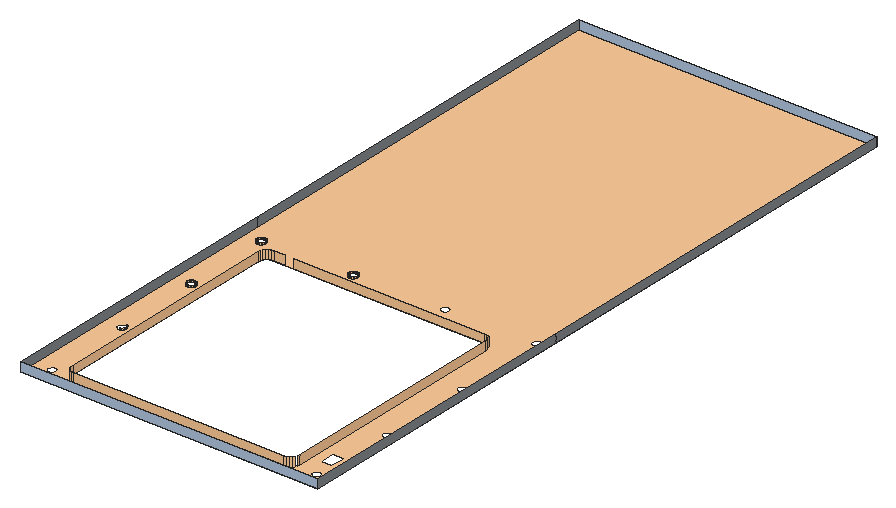
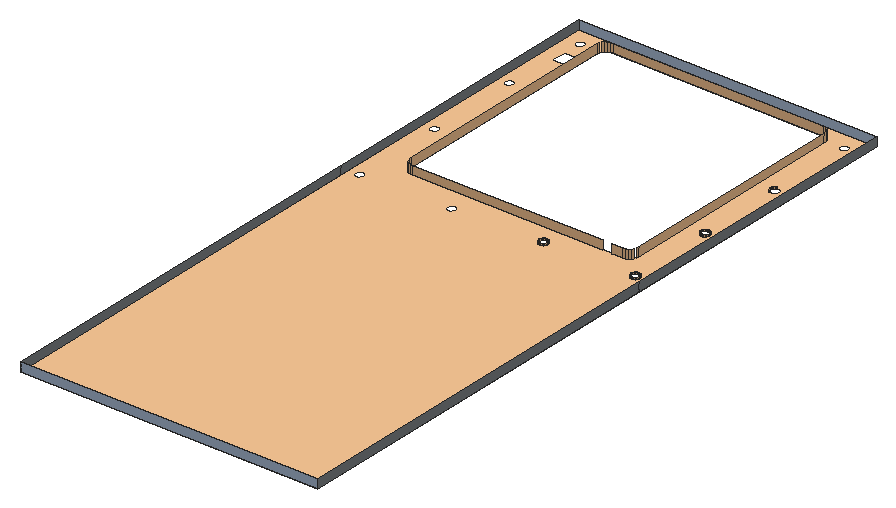
# SketchUp Ruby script. Lengths in inches.
U = 1.inch
M = Sketchup.active_model
def pt(a) = Geom::Point3d.new(a.map { |v| v * U })
def face(e, loops, mat)
  f = e.add_face(loops[0].map { |a| pt(a) })
  loops[1..].each { |l| e.add_face(l.map { |a| pt(a) }).erase! }
  f.material = f.back_material = mat if mat
  f
end
# faces: each face lists its corners as indices into pts; further lists are holes
def faces(e, pts, list, mat = nil) = list.each { |f| face(e, (f[0].is_a?(Array) ? f : [f]).map { |l| l.map { |i| pts[i] } }, mat) }
# xy, xz, yz: faces in a plane at the given z, y or x. An outline is a flat list of corners, or four numbers for a rectangle; further outlines are holes
def ring(l) = l.size == 4 ? [[l[0], l[1]], [l[2], l[1]], [l[2], l[3]], [l[0], l[3]]] : l.each_slice(2).to_a
def flat(e, list, mat, &to3) = list.each { |f| face(e, (f[0].is_a?(Array) ? f : [f]).map { |l| ring(l).map { |u, v| to3.(u, v) } }, mat) }
def xy(e, z, list, mat = nil) = flat(e, list, mat) { |x, y| [x, y, z] }
def xz(e, y, list, mat = nil) = flat(e, list, mat) { |x, z| [x, y, z] }
def yz(e, x, list, mat = nil) = flat(e, list, mat) { |y, z| [x, y, z] }
def lines(e, pts, list) = list.each { |a, b| e.add_line(pt(pts[a]), pt(pts[b])) }
# prism: a flat outline (further loops are holes) pulled along v
def prism(e, loops, v, mat = nil)
  f = face(e, loops, mat); d = Geom::Vector3d.new(v.map { |x| x * U })
  f.pushpull(f.normal.samedirection?(d) ? d.length : -d.length)
end
def box(e, o, s, mat = nil) = prism(e, [[o, [o[0] + s[0], o[1], o[2]], [o[0] + s[0], o[1] + s[1], o[2]], [o[0], o[1] + s[1], o[2]]]], [0, 0, s[2]], mat)
def at(x, y, z, deg = 0) = Geom::Transformation.translation(pt([x, y, z])) * Geom::Transformation.rotation(ORIGIN, Z_AXIS, deg.degrees)
def axes(o, x, y, z) = Geom::Transformation.new([*x, 0, *y, 0, *z, 0, *pt(o).to_a, 1])
def part(name) = M.definitions.add(name)
# library, detail: a bought-in or finely detailed component or shape, given as its bounding box
def library(name, o, s) = part(name).tap { |d| box(d.entities, o, s) }
def detail(e, o, s) = box(e.add_group.entities, o, s)
def put(e, d, t, mat = nil) = e.add_instance(d, t).tap { |i| i.material = mat if mat }
def group(e, t, mat = nil) = e.add_group.tap { |g| g.transformation = t; g.material = mat if mat }.entities
root = M.entities
M.materials.add("[0099_LightSteelBlue]").color = [176, 196, 222]
M.materials.add("[Blacktop Old 01]").color = [132, 136, 139]
M.materials.add("[Color C02]").color = [255, 204, 153]
xy(root,372,[[[0,130.0625,203.78,607.58],[30,138.625,173.78,138.625,175.61,138.79,177.11,139.29,178.28,140.125,179.11,141.29,179.61,142.79,179.78,144.625,179.78,303.17,179.61,305,179.11,306.5,178.28,307.67,177.11,308.5,175.61,309,173.78,309.17,30,309.17,28.17,309,26.67,308.5,25.5,307.67,24.67,306.5,24.17,305,24,303.17,24,144.625,24.17,142.79,24.67,141.29,25.5,140.125,26.67,139.29,28.17,138.79],[186.48,154.03,194.3,164.47],[196.29,195.4,197.07,195.47,197.81,195.74,198.45,196.19,198.95,196.78,199.29,197.49,199.42,198.27,199.36,199.05,199.09,199.78,198.64,200.42,198.04,200.93,197.33,201.26,196.56,201.4,195.78,201.33,195.04,201.0625,194.4,200.61,193.9,200.01,193.57,199.3,193.43,198.53,193.5,197.75,193.76,197.02,194.21,196.375,194.8125,195.87,195.52,195.54],[196.29,259.4,197.07,259.47,197.81,259.74,198.45,260.19,198.95,260.78,199.29,261.49,199.42,262.27,199.36,263.05,199.09,263.78,198.64,264.42,198.04,264.93,197.33,265.26,196.56,265.4,195.78,265.33,195.04,265.0625,194.4,264.61,193.9,264.01,193.57,263.3,193.43,262.53,193.5,261.75,193.76,261.02,194.21,260.375,194.8125,259.87,195.52,259.54],[193.29,138.77,194.07,138.83,194.81,139.1,195.45,139.55,195.95,140.15,196.29,140.86,196.42,141.63,196.36,142.41,196.09,143.15,195.64,143.79,195.04,144.29,194.33,144.625,193.56,144.76,192.78,144.69,192.04,144.43,191.4,143.98,190.9,143.38,190.57,142.67,190.43,141.9,190.5,141.12,190.76,140.38,191.21,139.74,191.8125,139.23,192.52,138.9],[11.87,139.23,12.65,139.3,13.38,139.57,14.02,140.02,14.53,140.62,14.86,141.33,15,142.1,14.93,142.88,14.66,143.61,14.21,144.26,13.61,144.76,12.9,145.09,12.13,145.23,11.35,145.16,10.62,144.89,9.98,144.44,9.47,143.85,9.14,143.14,9,142.36,9.07,141.58,9.34,140.85,9.79,140.21,10.39,139.7,11.1,139.37],[11.87,198.88,12.65,198.95,13.38,199.21,14.02,199.66,14.53,200.26,14.86,200.97,15,201.74,14.93,202.52,14.66,203.26,14.21,203.9,13.61,204.41,12.9,204.74,12.13,204.875,11.35,204.81,10.62,204.54,9.98,204.09,9.47,203.49,9.14,202.78,9,202.01,9.07,201.23,9.34,200.49,9.79,199.85,10.39,199.35,11.1,199.02],[11.87,258.53,12.65,258.59,13.38,258.86,14.02,259.31,14.53,259.91,14.86,260.62,15,261.39,14.93,262.17,14.66,262.91,14.21,263.55,13.61,264.05,12.9,264.38,12.13,264.52,11.35,264.45,10.62,264.19,9.98,263.74,9.47,263.14,9.14,262.43,9,261.66,9.07,260.875,9.34,260.14,9.79,259.5,10.39,258.99,11.1,258.66],[134.82,321.66,135.6,321.73,136.33,321.99,136.98,322.44,137.48,323.04,137.8125,323.75,137.95,324.52,137.88,325.3,137.61,326.04,137.16,326.68,136.56,327.18,135.86,327.52,135.08,327.65,134.3,327.58,133.57,327.32,132.93,326.87,132.42,326.27,132.09,325.56,131.95,324.79,132.02,324.01,132.29,323.27,132.74,322.63,133.34,322.125,134.05,321.79],[11.87,318.17,12.65,318.24,13.38,318.51,14.02,318.96,14.53,319.55,14.86,320.26,15,321.04,14.93,321.82,14.66,322.55,14.21,323.19,13.61,323.7,12.9,324.03,12.13,324.17,11.35,324.1,10.62,323.83,9.98,323.38,9.47,322.78,9.14,322.07,9,321.3,9.07,320.52,9.34,319.79,9.79,319.14,10.39,318.64,11.1,318.31],[73.34,319.91,74.12,319.98,74.86,320.25,75.5,320.7,76,321.3,76.34,322.01,76.47,322.78,76.4,323.56,76.14,324.29,75.6875,324.9375,75.09,325.44,74.38,325.77,73.61,325.91,72.83,325.84,72.09,325.57,71.45,325.125,70.95,324.53,70.61,323.82,70.48,323.05,70.55,322.27,70.8125,321.53,71.26,320.89,71.86,320.38,72.57,320.05],[196.29,323.4,197.07,323.47,197.81,323.74,198.45,324.19,198.95,324.78,199.29,325.49,199.42,326.27,199.36,327.05,199.09,327.78,198.64,328.42,198.04,328.93,197.33,329.26,196.56,329.4,195.78,329.33,195.04,329.0625,194.4,328.61,193.9,328.01,193.57,327.3,193.43,326.53,193.5,325.75,193.76,325.02,194.21,324.375,194.8125,323.87,195.52,323.54]]],"[Color C02]")
xz(root,130.0625,[[0,372,203.78,378]],"[0099_LightSteelBlue]")
xz(root,138.625,[[30,372,173.78,378]],"[Color C02]")
xz(root,309.17,[[30,372,37.58,378],[43.58,372,173.78,378]],"[Color C02]")
xz(root,607.58,[[0,372,203.78,378]],"[0099_LightSteelBlue]")
yz(root,0,[[130.0625,372,333.17,378],[333.17,372,607.58,378]],"[Blacktop Old 01]")
yz(root,24,[[144.625,372,303.17,378]],"[Color C02]")
yz(root,179.78,[[144.625,372,303.17,378]],"[Color C02]")
yz(root,203.78,[[130.0625,372,333.17,378],[333.17,372,607.58,378]],"[Blacktop Old 01]")
p = [[28.17,138.79,372],[28.17,138.79,378],[30,138.625,378],[30,138.625,372],[175.61,138.79,378],[175.61,138.79,372],
  [173.78,138.625,372],[173.78,138.625,378],[26.67,139.29,372],[26.67,139.29,378],[177.11,139.29,378],[177.11,139.29,372],
  [25.5,140.125,372],[25.5,140.125,378],[178.28,140.125,378],[178.28,140.125,372],[24.67,141.29,372],[24.67,141.29,378],
  [179.11,141.29,378],[179.11,141.29,372],[24,144.625,372],[24,144.625,378],[24.17,142.79,378],[24.17,142.79,372],
  [179.78,144.625,378],[179.78,144.625,372],[179.61,142.79,372],[179.61,142.79,378],[13.38,199.21,372],[12.65,198.95,372],
  [12.65,198.95,373],[13.38,199.21,373],[14.02,199.66,372],[14.02,199.66,373],[14.53,200.26,372],[14.53,200.26,373],
  [14.86,200.97,372],[14.86,200.97,373],[15,201.74,372],[15,201.74,373],[14.93,202.52,372],[14.93,202.52,373],
  [14.66,203.26,372],[14.66,203.26,373],[14.21,203.9,372],[14.21,203.9,373],[13.61,204.41,372],[13.61,204.41,373],
  [11.87,258.53,372],[11.1,258.66,372],[11.1,258.66,373],[11.87,258.53,373],[12.65,258.59,372],[12.65,258.59,373],
  [13.38,258.86,372],[13.38,258.86,373],[10.39,258.99,372],[10.39,258.99,373],[14.02,259.31,372],[14.02,259.31,373],
  [9.79,259.5,372],[9.79,259.5,373],[14.53,259.91,372],[14.53,259.91,373],[9.34,260.14,372],[9.34,260.14,373],
  [14.86,260.62,372],[14.86,260.62,373],[9.07,260.875,372],[9.07,260.875,373],[15,261.39,372],[15,261.39,373],
  [9,261.66,372],[9,261.66,373],[14.93,262.17,372],[14.93,262.17,373],[9.14,262.43,372],[9.14,262.43,373],
  [14.66,262.91,372],[14.66,262.91,373],[9.47,263.14,372],[9.47,263.14,373],[14.21,263.55,372],[14.21,263.55,373],
  [9.98,263.74,372],[9.98,263.74,373],[13.61,264.05,372],[13.61,264.05,373],[10.62,264.19,372],[10.62,264.19,373],
  [12.9,264.38,372],[12.9,264.38,373],[11.35,264.45,372],[11.35,264.45,373],[12.13,264.52,372],[12.13,264.52,373],
  [24,303.17,378],[24,303.17,372],[24.17,305,372],[24.17,305,378],[179.78,303.17,372],[179.78,303.17,378],
  [179.61,305,378],[179.61,305,372],[24.67,306.5,378],[24.67,306.5,372],[25.5,307.67,372],[25.5,307.67,378],
  [179.11,306.5,372],[179.11,306.5,378],[178.28,307.67,378],[178.28,307.67,372],[26.67,308.5,372],[26.67,308.5,378],
  [177.11,308.5,378],[177.11,308.5,372],[28.17,309,372],[28.17,309,378],[175.61,309,378],[175.61,309,372],
  [30,309.17,372],[30,309.17,378],[173.78,309.17,378],[173.78,309.17,372],[11.87,318.17,372],[11.1,318.31,372],
  [11.1,318.31,373],[11.87,318.17,373],[12.65,318.24,372],[12.65,318.24,373],[13.38,318.51,372],[13.38,318.51,373],
  [10.39,318.64,372],[10.39,318.64,373],[14.02,318.96,372],[14.02,318.96,373],[9.79,319.14,372],[9.79,319.14,373],
  [14.53,319.55,372],[14.53,319.55,373],[9.34,319.79,372],[9.34,319.79,373],[14.86,320.26,372],[14.86,320.26,373],
  [9.07,320.52,372],[9.07,320.52,373],[73.34,319.91,372],[72.57,320.05,372],[72.57,320.05,373],[73.34,319.91,373],
  [74.12,319.98,372],[74.12,319.98,373],[74.86,320.25,372],[74.86,320.25,373],[71.86,320.38,372],[71.86,320.38,373],
  [75.5,320.7,372],[75.5,320.7,373],[15,321.04,372],[15,321.04,373],[71.26,320.89,372],[71.26,320.89,373],
  [9,321.3,372],[9,321.3,373],[76,321.3,372],[76,321.3,373],[70.8125,321.53,372],[70.8125,321.53,373],
  [14.93,321.82,372],[14.93,321.82,373],[9.14,322.07,372],[9.14,322.07,373],[76.34,322.01,372],[76.34,322.01,373],
  [70.55,322.27,372],[70.55,322.27,373],[14.66,322.55,372],[14.66,322.55,373],[76.47,322.78,372],[76.47,322.78,373],
  [9.47,322.78,372],[9.47,322.78,373],[70.48,323.05,372],[70.48,323.05,373],[14.21,323.19,372],[14.21,323.19,373],
  [9.98,323.38,372],[9.98,323.38,373],[76.4,323.56,372],[76.4,323.56,373],[70.61,323.82,372],[70.61,323.82,373],
  [13.61,323.7,372],[13.61,323.7,373],[10.62,323.83,372],[10.62,323.83,373],[76.14,324.29,372],[76.14,324.29,373],
  [12.9,324.03,372],[12.9,324.03,373],[11.35,324.1,372],[11.35,324.1,373],[70.95,324.53,372],[70.95,324.53,373],
  [12.13,324.17,372],[12.13,324.17,373],[75.6875,324.9375,372],[75.6875,324.9375,373],[71.45,325.125,372],[71.45,325.125,373],
  [75.09,325.44,372],[75.09,325.44,373],[72.09,325.57,372],[72.09,325.57,373],[74.38,325.77,372],[74.38,325.77,373],
  [72.83,325.84,372],[72.83,325.84,373],[73.61,325.91,372],[73.61,325.91,373]]
faces(root,p,[[0,1,2,3],[4,5,6,7],[8,9,1,0],[10,11,5,4],[12,13,9,8],[14,15,11,10],[16,17,13,12],[18,19,15,14],
  [20,21,22,23],[24,25,26,27],[28,29,30,31],[32,28,31,33],[34,32,33,35],[36,34,35,37],[38,36,37,39],[40,38,39,41],
  [42,40,41,43],[44,42,43,45],[46,44,45,47],[48,49,50,51],[52,48,51,53],[54,52,53,55],[49,56,57,50],[58,54,55,59],
  [56,60,61,57],[62,58,59,63],[60,64,65,61],[66,62,63,67],[64,68,69,65],[70,66,67,71],[68,72,73,69],[74,70,71,75],
  [72,76,77,73],[78,74,75,79],[76,80,81,77],[82,78,79,83],[80,84,85,81],[86,82,83,87],[84,88,89,85],[90,86,87,91],
  [88,92,93,89],[94,90,91,95],[92,94,95,93],[96,97,98,99],[100,101,102,103],[104,105,106,107],[108,109,110,111],[107,106,112,113],
  [111,110,114,115],[113,112,116,117],[115,114,118,119],[117,116,120,121],[119,118,122,123],[124,125,126,127],[128,124,127,129],[130,128,129,131],
  [125,132,133,126],[134,130,131,135],[132,136,137,133],[138,134,135,139],[136,140,141,137],[142,138,139,143],[140,144,145,141],[146,147,148,149],
  [150,146,149,151],[152,150,151,153],[147,154,155,148],[156,152,153,157],[158,142,143,159],[154,160,161,155],[144,162,163,145],[164,156,157,165],
  [160,166,167,161],[168,158,159,169],[162,170,171,163],[172,164,165,173],[166,174,175,167],[176,168,169,177],[178,172,173,179],[170,180,181,171],
  [174,182,183,175],[184,176,177,185],[180,186,187,181],[188,178,179,189],[182,190,191,183],[192,184,185,193],[186,194,195,187],[196,188,189,197],
  [198,192,193,199],[194,200,201,195],[190,202,203,191],[204,198,199,205],[200,204,205,201],[206,196,197,207],[202,208,209,203],[210,206,207,211],
  [208,212,213,209],[214,210,211,215],[212,216,217,213],[216,218,219,217],[218,214,215,219]],"[Color C02]")
